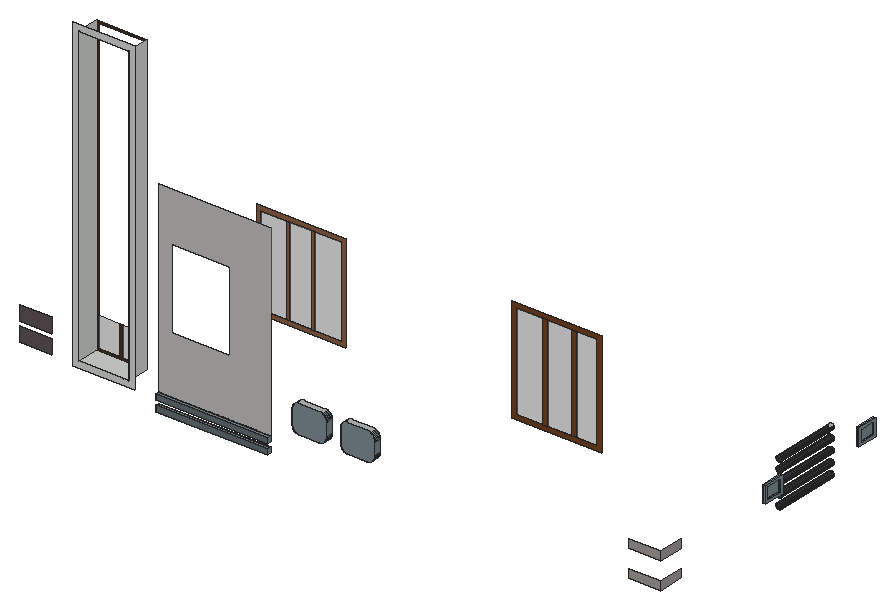
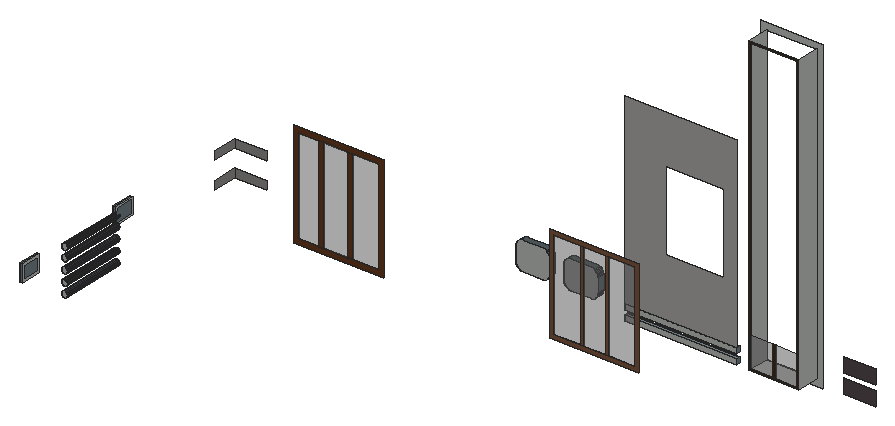
# SketchUp Ruby script. Lengths in inches.
U = 1.inch
M = Sketchup.active_model
def pt(a) = Geom::Point3d.new(a.map { |v| v * U })
def face(e, loops, mat)
  f = e.add_face(loops[0].map { |a| pt(a) })
  loops[1..].each { |l| e.add_face(l.map { |a| pt(a) }).erase! }
  f.material = f.back_material = mat if mat
  f
end
# faces: each face lists its corners as indices into pts; further lists are holes
def faces(e, pts, list, mat = nil) = list.each { |f| face(e, (f[0].is_a?(Array) ? f : [f]).map { |l| l.map { |i| pts[i] } }, mat) }
# xy, xz, yz: faces in a plane at the given z, y or x. An outline is a flat list of corners, or four numbers for a rectangle; further outlines are holes
def ring(l) = l.size == 4 ? [[l[0], l[1]], [l[2], l[1]], [l[2], l[3]], [l[0], l[3]]] : l.each_slice(2).to_a
def flat(e, list, mat, &to3) = list.each { |f| face(e, (f[0].is_a?(Array) ? f : [f]).map { |l| ring(l).map { |u, v| to3.(u, v) } }, mat) }
def xy(e, z, list, mat = nil) = flat(e, list, mat) { |x, y| [x, y, z] }
def xz(e, y, list, mat = nil) = flat(e, list, mat) { |x, z| [x, y, z] }
def yz(e, x, list, mat = nil) = flat(e, list, mat) { |y, z| [x, y, z] }
def lines(e, pts, list) = list.each { |a, b| e.add_line(pt(pts[a]), pt(pts[b])) }
# prism: a flat outline (further loops are holes) pulled along v
def prism(e, loops, v, mat = nil)
  f = face(e, loops, mat); d = Geom::Vector3d.new(v.map { |x| x * U })
  f.pushpull(f.normal.samedirection?(d) ? d.length : -d.length)
end
def box(e, o, s, mat = nil) = prism(e, [[o, [o[0] + s[0], o[1], o[2]], [o[0] + s[0], o[1] + s[1], o[2]], [o[0], o[1] + s[1], o[2]]]], [0, 0, s[2]], mat)
def at(x, y, z, deg = 0) = Geom::Transformation.translation(pt([x, y, z])) * Geom::Transformation.rotation(ORIGIN, Z_AXIS, deg.degrees)
def axes(o, x, y, z) = Geom::Transformation.new([*x, 0, *y, 0, *z, 0, *pt(o).to_a, 1])
def part(name) = M.definitions.add(name)
# library, detail: a bought-in or finely detailed component or shape, given as its bounding box
def library(name, o, s) = part(name).tap { |d| box(d.entities, o, s) }
def detail(e, o, s) = box(e.add_group.entities, o, s)
def put(e, d, t, mat = nil) = e.add_instance(d, t).tap { |i| i.material = mat if mat }
def group(e, t, mat = nil) = e.add_group.tap { |g| g.transformation = t; g.material = mat if mat }.entities
root = M.entities
M.materials.add("[Asphalt New]").color = [89, 79, 82]
M.materials.add("[Basic Tile]").color = [203, 206, 202]
M.materials.add("[Brick Tumbled]").color = [186, 182, 182]
M.materials.add("[Concrete Aggregate Smoke]").color = [154, 150, 148]
M.materials.add("[Formica Laminate Dark]1").color = [65, 69, 79]
M.materials.add("[Formica Speckled Grey]").color = [120, 135, 142]
M.materials.add("[Formica Speckled Grey]1").color = [94, 105, 111]
M.materials.add("[Translucent Glass Gray]").color = [128, 128, 128]
M.materials["[Translucent Glass Gray]"].alpha = 0.5
M.materials.add("[Wood Floor]").color = [71, 48, 28]
M.materials.add("[Wood Veneer 01]1").color = [109, 63, 33]
M.materials.add("[Wood Veneer 02]").color = [137, 92, 65]
xy(root,405.57,[[523.06,696.47,716.67,703.09]],"[Formica Speckled Grey]")
xy(root,414.9375,[[523.06,696.47,716.67,703.09]],"[Formica Speckled Grey]")
xy(root,423.19,[[523.06,696.47,716.67,703.09]],"[Formica Speckled Grey]")
xy(root,432.42,[[385.1,703.09,471.56,741.66]],"[Basic Tile]")
xy(root,432.5625,[[523.06,696.47,716.67,703.09]],"[Formica Speckled Grey]")
xy(root,440.05,[[753.68,719.27,788.14,730.52],[837.48,719.27,870.82,730.52]],"[Formica Speckled Grey]")
xy(root,449.17,[[1370.47,951.61,1374.84,988.05],[1370.47,1153.55,1374.84,1189.99]],"[Formica Speckled Grey]")
xy(root,452.5625,[[1370.47,955.01,1374.84,984.66],[1370.47,1156.95,1374.84,1186.59]],"[Formica Speckled Grey]")
xy(root,474.52,[[1370.47,955.01,1374.84,984.66],[1370.47,1156.95,1374.84,1186.59]],"[Formica Speckled Grey]")
xy(root,477.92,[[1370.47,951.61,1374.84,988.05],[1370.47,1153.55,1374.84,1189.99]],"[Formica Speckled Grey]")
xz(root,696.47,[[523.06,405.57,716.67,414.9375],[523.06,423.19,716.67,432.5625]],"[Formica Speckled Grey]1")
xz(root,703.09,[[282.77,425.33,338.2,450.58],[282.77,458.7,338.2,483.95]],"[Asphalt New]")
xz(root,703.09,[[523.06,405.57,716.67,414.9375],[[374.08,421.4,482.58,954.84],[385.1,432.42,471.56,943.81]],[523.06,423.19,716.67,432.5625]],"[Basic Tile]")
xz(root,703.09,[[[523.06,432.5625,716.67,754.78],[546.1,532.7,646.79,670.32]]],"[Brick Tumbled]")
xz(root,719.27,[[753.68,440.05,788.14,440.05,789.8125,440.16,791.46,440.49,793.05,441.03,794.55,441.77,795.95,442.71,797.21,443.8125,798.32,445.07,799.25,446.47,799.99,447.97,800.53,449.5625,800.86,451.21,800.97,452.88,800.97,476.1,800.86,477.72,800.54,479.31,800.02,480.84,799.31,482.3,798.41,483.64,797.34,484.86,796.12,485.93,794.77,486.83,793.32,487.55,791.78,488.07,790.19,488.39,788.57,488.49,753.6875,488.49,752.04,488.38,750.43,488.0625,748.87,487.53,747.39,486.8,746.02,485.89,744.78,484.8,743.69,483.56,742.78,482.2,742.05,480.72,741.52,479.16,741.2,477.54,741.09,475.9,741.09,452.64,741.2,451,741.52,449.38,742.05,447.82,742.78,446.35,743.69,444.98,744.78,443.74,746.02,442.65,747.38,441.74,748.86,441.01,750.42,440.48,752.03,440.16],[837.48,440.05,870.82,440.05,872.63,440.17,874.42,440.53,876.14,441.11,877.77,441.92,879.28,442.93,880.65,444.125,881.85,445.49,882.86,447,883.66,448.63,884.24,450.36,884.6,452.14,884.72,453.95,884.72,474.16,884.59,476.03,884.23,477.87,883.625,479.64,882.8,481.32,881.76,482.88,880.52,484.29,879.11,485.53,877.55,486.57,875.87,487.4,874.09,488,872.25,488.37,870.38,488.49,837.19,488.49,835.58,488.39,833.99,488.07,832.46,487.55,831.02,486.84,829.67,485.94,828.46,484.875,827.39,483.66,826.5,482.32,825.78,480.87,825.26,479.34,824.95,477.76,824.84,476.14,824.84,452.69,824.95,451.04,825.27,449.42,825.8,447.85,826.53,446.37,827.45,445,828.54,443.76,829.79,442.67,831.16,441.75,832.64,441.02,834.21,440.48,835.83,440.16]],"[Formica Speckled Grey]")
xz(root,730.52,[[753.68,440.05,752.03,440.16,750.42,440.48,748.86,441.01,747.38,441.74,746.02,442.65,744.78,443.74,743.69,444.98,742.78,446.35,742.05,447.82,741.52,449.38,741.2,451,741.09,452.64,741.09,475.9,741.2,477.54,741.52,479.16,742.05,480.72,742.78,482.2,743.69,483.56,744.78,484.8,746.02,485.89,747.39,486.8,748.87,487.53,750.43,488.0625,752.04,488.38,753.6875,488.49,788.57,488.49,790.19,488.39,791.78,488.07,793.32,487.55,794.77,486.83,796.12,485.93,797.34,484.86,798.41,483.64,799.31,482.3,800.02,480.84,800.54,479.31,800.86,477.72,800.97,476.1,800.97,452.88,800.86,451.21,800.53,449.5625,799.99,447.97,799.25,446.47,798.32,445.07,797.21,443.8125,795.95,442.71,794.55,441.77,793.05,441.03,791.46,440.49,789.8125,440.16,788.14,440.05],[837.48,440.05,835.83,440.16,834.21,440.48,832.64,441.02,831.16,441.75,829.79,442.67,828.54,443.76,827.45,445,826.53,446.37,825.8,447.85,825.27,449.42,824.95,451.04,824.84,452.69,824.84,476.14,824.95,477.76,825.26,479.34,825.78,480.87,826.5,482.32,827.39,483.66,828.46,484.875,829.67,485.94,831.02,486.84,832.46,487.55,833.99,488.07,835.58,488.39,837.19,488.49,870.38,488.49,872.25,488.37,874.09,488,875.87,487.4,877.55,486.57,879.11,485.53,880.52,484.29,881.76,482.88,882.8,481.32,883.625,479.64,884.23,477.87,884.59,476.03,884.72,474.16,884.72,453.95,884.6,452.14,884.24,450.36,883.66,448.63,882.86,447,881.85,445.49,880.65,444.125,879.28,442.93,877.77,441.92,876.14,441.11,874.42,440.53,872.63,440.17,870.82,440.05]],"[Basic Tile]")
xz(root,730.52,[[1314.99,410.47,1370.47,425.22],[1314.99,456.66,1370.47,471.41]],"[Concrete Aggregate Smoke]")
xz(root,741.66,[[387.85,435.17,425.21,487.63],[430.65,435.17,468.81,487.63]],"[Translucent Glass Gray]")
xz(root,741.66,[[[385.1,432.42,471.56,943.81],[387.85,435.17,468.81,941.07]],[425.21,435.17,430.65,487.63]],"[Wood Floor]")
xz(root,898.23,[[987.57,475.01,1032.05,640.23],[1039.98,475.01,1082.49,640.23],[1090.42,475.01,1125.29,640.23],[544.07,481.83,588.26,635.98],[594.65,481.83,631.26,635.98],
  [637.65,481.83,683.83,635.98]],"[Translucent Glass Gray]")
xz(root,898.23,[[[978.99,466.43,1133.86,648.81],[987.57,475.01,1125.29,640.23]],[1032.05,475.01,1039.98,640.23],[1082.49,475.01,1090.42,640.23]],"[Wood Veneer 01]1")
xz(root,898.23,[[[536.84,474.6,691.07,643.21],[544.07,481.83,683.83,635.98]],[588.26,481.83,594.65,635.98],[631.26,481.83,637.65,635.98]],"[Wood Veneer 02]")
xz(root,951.61,[[1370.47,449.17,1374.84,477.92]],"[Formica Speckled Grey]")
xz(root,955.01,[[1370.47,452.5625,1374.84,474.52]],"[Formica Speckled Grey]")
xz(root,984.66,[[1370.47,452.5625,1374.84,474.52]],"[Formica Speckled Grey]")
xz(root,988.05,[[1370.47,449.17,1374.84,477.92]],"[Formica Speckled Grey]")
xz(root,1125.19,[[1349.2,405.1,1347.875,405.28,1346.64,405.79,1345.58,406.61,1344.76,407.67,1344.25,408.9,1344.08,410.23,1344.25,411.56,1344.76,412.79,1345.58,413.85,1346.64,414.67,1347.875,415.18,1349.2,415.35,1350.53,415.18,1351.77,414.67,1352.83,413.85,1353.64,412.79,1354.15,411.56,1354.33,410.23,1354.15,408.9,1353.64,407.67,1352.83,406.61,1351.77,405.79,1350.53,405.28],[1349.2,423.29,1347.875,423.47,1346.64,423.98,1345.58,424.79,1344.76,425.85,1344.25,427.09,1344.08,428.42,1344.25,429.74,1344.76,430.98,1345.58,432.04,1346.64,432.86,1347.875,433.37,1349.2,433.54,1350.53,433.37,1351.77,432.86,1352.83,432.04,1353.64,430.98,1354.15,429.74,1354.33,428.42,1354.15,427.09,1353.64,425.85,1352.83,424.79,1351.77,423.98,1350.53,423.47],[1349.2,442.67,1347.875,442.84,1346.64,443.35,1345.58,444.17,1344.76,445.23,1344.25,446.47,1344.08,447.79,1344.25,449.12,1344.76,450.35,1345.58,451.42,1346.64,452.23,1347.875,452.74,1349.2,452.92,1350.53,452.74,1351.77,452.23,1352.83,451.42,1353.64,450.35,1354.15,449.12,1354.33,447.79,1354.15,446.47,1353.64,445.23,1352.83,444.17,1351.77,443.35,1350.53,442.84],[1349.2,461.48,1347.875,461.65,1346.64,462.17,1345.58,462.98,1344.76,464.04,1344.25,465.28,1344.08,466.6,1344.25,467.93,1344.76,469.17,1345.58,470.23,1346.64,471.04,1347.875,471.55,1349.2,471.73,1350.53,471.55,1351.77,471.04,1352.83,470.23,1353.64,469.17,1354.15,467.93,1354.33,466.6,1354.15,465.28,1353.64,464.04,1352.83,462.98,1351.77,462.17,1350.53,461.65],[1349.2,478.79,1347.875,478.97,1346.64,479.48,1345.58,480.29,1344.76,481.35,1344.25,482.59,1344.08,483.92,1344.25,485.24,1344.76,486.48,1345.58,487.54,1346.64,488.36,1347.875,488.87,1349.2,489.04,1350.53,488.87,1351.77,488.36,1352.83,487.54,1353.64,486.48,1354.15,485.24,1354.33,483.92,1354.15,482.59,1353.64,481.35,1352.83,480.29,1351.77,479.48,1350.53,478.97]],"[Basic Tile]")
xz(root,1153.55,[[1370.47,449.17,1374.84,477.92]],"[Formica Speckled Grey]")
xz(root,1156.95,[[1370.47,452.5625,1374.84,474.52]],"[Formica Speckled Grey]")
xz(root,1186.59,[[1370.47,452.5625,1374.84,474.52]],"[Formica Speckled Grey]")
xz(root,1189.99,[[1370.47,449.17,1374.84,477.92]],"[Formica Speckled Grey]")
yz(root,385.1,[[703.09,432.42,741.66,943.81]],"[Basic Tile]")
yz(root,471.56,[[703.09,432.42,741.66,943.81]],"[Basic Tile]")
yz(root,523.06,[[696.47,405.57,703.09,414.9375],[696.47,423.19,703.09,432.5625]],"[Formica Speckled Grey]")
yz(root,716.67,[[696.47,405.57,703.09,414.9375],[696.47,423.19,703.09,432.5625]],"[Formica Speckled Grey]")
yz(root,741.09,[[719.27,452.64,730.52,475.9]],"[Formica Speckled Grey]")
yz(root,800.97,[[719.27,452.88,730.52,476.1]],"[Formica Speckled Grey]")
yz(root,824.84,[[719.27,452.69,730.52,476.14]],"[Formica Speckled Grey]")
yz(root,884.72,[[719.27,453.95,730.52,474.16]],"[Formica Speckled Grey]")
yz(root,1370.47,[[[951.61,449.17,988.05,477.92],[955.01,452.5625,984.66,474.52]],[[1153.55,449.17,1189.99,477.92],[1156.95,452.5625,1186.59,474.52]]],"[Basic Tile]")
yz(root,1370.47,[[730.52,410.47,774.21,425.22],[730.52,456.66,774.21,471.41]],"[Concrete Aggregate Smoke]")
yz(root,1370.47,[[955.01,452.5625,984.66,474.52],[1156.95,452.5625,1186.59,474.52]],"[Formica Speckled Grey]")
yz(root,1374.84,[[[951.61,449.17,988.05,477.92],[955.01,452.5625,984.66,474.52]],[[1153.55,449.17,1189.99,477.92],[1156.95,452.5625,1186.59,474.52]]],"[Formica Speckled Grey]")
p = [[1347.875,1125.19,405.28],[1349.2,1125.19,405.1],[1349.2,1012.73,405.1],[1347.875,1012.73,405.28],[1350.53,1125.19,405.28],[1350.53,1012.73,405.28],
  [1346.64,1125.19,405.79],[1346.64,1012.73,405.79],[1351.77,1125.19,405.79],[1351.77,1012.73,405.79],[1345.58,1125.19,406.61],[1345.58,1012.73,406.61],
  [1352.83,1125.19,406.61],[1352.83,1012.73,406.61],[1344.76,1125.19,407.67],[1344.76,1012.73,407.67],[1353.64,1125.19,407.67],[1353.64,1012.73,407.67],
  [1344.25,1125.19,408.9],[1344.25,1012.73,408.9],[1354.15,1125.19,408.9],[1354.15,1012.73,408.9],[1344.08,1125.19,410.23],[1344.08,1012.73,410.23],
  [1354.33,1125.19,410.23],[1354.33,1012.73,410.23],[1344.25,1125.19,411.56],[1344.25,1012.73,411.56],[1354.15,1125.19,411.56],[1354.15,1012.73,411.56],
  [1344.76,1125.19,412.79],[1344.76,1012.73,412.79],[1353.64,1125.19,412.79],[1353.64,1012.73,412.79],[1345.58,1125.19,413.85],[1345.58,1012.73,413.85],
  [1352.83,1125.19,413.85],[1352.83,1012.73,413.85],[1346.64,1125.19,414.67],[1346.64,1012.73,414.67],[1351.77,1125.19,414.67],[1351.77,1012.73,414.67],
  [1347.875,1125.19,415.18],[1347.875,1012.73,415.18],[1350.53,1125.19,415.18],[1350.53,1012.73,415.18],[1349.2,1125.19,415.35],[1349.2,1012.73,415.35],
  [1347.875,1125.19,423.47],[1349.2,1125.19,423.29],[1349.2,1012.73,423.29],[1347.875,1012.73,423.47],[1350.53,1125.19,423.47],[1350.53,1012.73,423.47],
  [1346.64,1125.19,423.98],[1346.64,1012.73,423.98],[1351.77,1125.19,423.98],[1351.77,1012.73,423.98],[1345.58,1125.19,424.79],[1345.58,1012.73,424.79],
  [1352.83,1125.19,424.79],[1352.83,1012.73,424.79],[1344.76,1125.19,425.85],[1344.76,1012.73,425.85],[1353.64,1125.19,425.85],[1353.64,1012.73,425.85],
  [1344.25,1125.19,427.09],[1344.25,1012.73,427.09],[1354.15,1125.19,427.09],[1354.15,1012.73,427.09],[1344.08,1125.19,428.42],[1344.08,1012.73,428.42],
  [1354.33,1125.19,428.42],[1354.33,1012.73,428.42],[1344.25,1125.19,429.74],[1344.25,1012.73,429.74],[1354.15,1125.19,429.74],[1354.15,1012.73,429.74],
  [1344.76,1125.19,430.98],[1344.76,1012.73,430.98],[1353.64,1125.19,430.98],[1353.64,1012.73,430.98],[1345.58,1125.19,432.04],[1345.58,1012.73,432.04],
  [1352.83,1125.19,432.04],[1352.83,1012.73,432.04],[1346.64,1125.19,432.86],[1346.64,1012.73,432.86],[1351.77,1125.19,432.86],[1351.77,1012.73,432.86],
  [1347.875,1125.19,433.37],[1347.875,1012.73,433.37],[1350.53,1125.19,433.37],[1350.53,1012.73,433.37],[1349.2,1125.19,433.54],[1349.2,1012.73,433.54],
  [752.03,730.52,440.16],[753.68,730.52,440.05],[753.68,719.27,440.05],[752.03,719.27,440.16],[788.14,730.52,440.05],[789.8125,730.52,440.16],
  [789.8125,719.27,440.16],[788.14,719.27,440.05],[835.83,730.52,440.16],[837.48,730.52,440.05],[837.48,719.27,440.05],[835.83,719.27,440.16],
  [870.82,730.52,440.05],[872.63,730.52,440.17],[872.63,719.27,440.17],[870.82,719.27,440.05],[750.42,730.52,440.48],[750.42,719.27,440.48],
  [791.46,730.52,440.49],[791.46,719.27,440.49],[834.21,730.52,440.48],[834.21,719.27,440.48],[874.42,730.52,440.53],[874.42,719.27,440.53],
  [748.86,730.52,441.01],[748.86,719.27,441.01],[793.05,730.52,441.03],[793.05,719.27,441.03],[832.64,730.52,441.02],[832.64,719.27,441.02],
  [876.14,730.52,441.11],[876.14,719.27,441.11],[747.38,730.52,441.74],[747.38,719.27,441.74],[794.55,730.52,441.77],[794.55,719.27,441.77],
  [831.16,730.52,441.75],[831.16,719.27,441.75],[877.77,730.52,441.92],[877.77,719.27,441.92],[746.02,730.52,442.65],[746.02,719.27,442.65],
  [829.79,730.52,442.67],[829.79,719.27,442.67],[795.95,730.52,442.71],[795.95,719.27,442.71],[879.28,730.52,442.93],[879.28,719.27,442.93],
  [744.78,730.52,443.74],[744.78,719.27,443.74],[797.21,730.52,443.8125],[797.21,719.27,443.8125],[828.54,730.52,443.76],[828.54,719.27,443.76],
  [1347.875,1125.19,442.84],[1349.2,1125.19,442.67],[1349.2,1012.73,442.67],[1347.875,1012.73,442.84],[1350.53,1125.19,442.84],[1350.53,1012.73,442.84],
  [1346.64,1125.19,443.35],[1346.64,1012.73,443.35],[1351.77,1125.19,443.35],[1351.77,1012.73,443.35],[880.65,730.52,444.125],[880.65,719.27,444.125],
  [1345.58,1125.19,444.17],[1345.58,1012.73,444.17],[1352.83,1125.19,444.17],[1352.83,1012.73,444.17],[743.69,730.52,444.98],[743.69,719.27,444.98],
  [798.32,730.52,445.07],[798.32,719.27,445.07],[827.45,730.52,445],[827.45,719.27,445],[881.85,730.52,445.49],[881.85,719.27,445.49],
  [1344.76,1125.19,445.23],[1344.76,1012.73,445.23],[1353.64,1125.19,445.23],[1353.64,1012.73,445.23],[742.78,730.52,446.35],[742.78,719.27,446.35],
  [826.53,730.52,446.37],[826.53,719.27,446.37],[799.25,730.52,446.47],[799.25,719.27,446.47],[1344.25,1125.19,446.47],[1344.25,1012.73,446.47],
  [1354.15,1125.19,446.47],[1354.15,1012.73,446.47],[882.86,730.52,447],[882.86,719.27,447],[742.05,730.52,447.82],[742.05,719.27,447.82],
  [825.8,730.52,447.85],[825.8,719.27,447.85],[799.99,730.52,447.97],[799.99,719.27,447.97],[1344.08,1125.19,447.79],[1344.08,1012.73,447.79],
  [1354.33,1125.19,447.79],[1354.33,1012.73,447.79],[883.66,730.52,448.63],[883.66,719.27,448.63],[741.52,730.52,449.38],[741.52,719.27,449.38],
  [1344.25,1125.19,449.12],[1344.25,1012.73,449.12],[1354.15,1125.19,449.12],[1354.15,1012.73,449.12],[825.27,730.52,449.42],[825.27,719.27,449.42],
  [800.53,730.52,449.5625],[800.53,719.27,449.5625],[884.24,730.52,450.36],[884.24,719.27,450.36],[1344.76,1125.19,450.35],[1344.76,1012.73,450.35],
  [1353.64,1125.19,450.35],[1353.64,1012.73,450.35],[741.2,730.52,451],[741.2,719.27,451],[824.95,730.52,451.04],[824.95,719.27,451.04],
  [800.86,730.52,451.21],[800.86,719.27,451.21],[884.6,730.52,452.14],[884.6,719.27,452.14],[1345.58,1125.19,451.42],[1345.58,1012.73,451.42],
  [1352.83,1125.19,451.42],[1352.83,1012.73,451.42],[741.09,730.52,452.64],[741.09,719.27,452.64],[824.84,730.52,452.69],[824.84,719.27,452.69],
  [800.97,730.52,452.88],[800.97,719.27,452.88],[1346.64,1125.19,452.23],[1346.64,1012.73,452.23],[1351.77,1125.19,452.23],[1351.77,1012.73,452.23],
  [884.72,730.52,453.95],[884.72,719.27,453.95],[1347.875,1125.19,452.74],[1347.875,1012.73,452.74],[1350.53,1125.19,452.74],[1350.53,1012.73,452.74],
  [1349.2,1125.19,452.92],[1349.2,1012.73,452.92],[1347.875,1125.19,461.65],[1349.2,1125.19,461.48],[1349.2,1012.73,461.48],[1347.875,1012.73,461.65],
  [1350.53,1125.19,461.65],[1350.53,1012.73,461.65],[1346.64,1125.19,462.17],[1346.64,1012.73,462.17],[1351.77,1125.19,462.17],[1351.77,1012.73,462.17],
  [1345.58,1125.19,462.98],[1345.58,1012.73,462.98],[1352.83,1125.19,462.98],[1352.83,1012.73,462.98],[1344.76,1125.19,464.04],[1344.76,1012.73,464.04],
  [1353.64,1125.19,464.04],[1353.64,1012.73,464.04],[1344.25,1125.19,465.28],[1344.25,1012.73,465.28],[1354.15,1125.19,465.28],[1354.15,1012.73,465.28],
  [1344.08,1125.19,466.6],[1344.08,1012.73,466.6],[1354.33,1125.19,466.6],[1354.33,1012.73,466.6],[1344.25,1125.19,467.93],[1344.25,1012.73,467.93],
  [1354.15,1125.19,467.93],[1354.15,1012.73,467.93],[1344.76,1125.19,469.17],[1344.76,1012.73,469.17],[1353.64,1125.19,469.17],[1353.64,1012.73,469.17],
  [1345.58,1125.19,470.23],[1345.58,1012.73,470.23],[1352.83,1125.19,470.23],[1352.83,1012.73,470.23],[1346.64,1125.19,471.04],[1346.64,1012.73,471.04],
  [1351.77,1125.19,471.04],[1351.77,1012.73,471.04],[1347.875,1125.19,471.55],[1347.875,1012.73,471.55],[1350.53,1125.19,471.55],[1350.53,1012.73,471.55],
  [1349.2,1125.19,471.73],[1349.2,1012.73,471.73],[884.72,730.52,474.16],[884.59,730.52,476.03],[884.59,719.27,476.03],[884.72,719.27,474.16],
  [741.2,730.52,477.54],[741.09,730.52,475.9],[741.09,719.27,475.9],[741.2,719.27,477.54],[884.23,730.52,477.87],[884.23,719.27,477.87],
  [800.97,730.52,476.1],[800.86,730.52,477.72],[800.86,719.27,477.72],[800.97,719.27,476.1],[824.95,730.52,477.76],[824.84,730.52,476.14],
  [824.84,719.27,476.14],[824.95,719.27,477.76],[741.52,730.52,479.16],[741.52,719.27,479.16],[800.54,730.52,479.31],[800.54,719.27,479.31],
  [825.26,730.52,479.34],[825.26,719.27,479.34],[883.625,730.52,479.64],[883.625,719.27,479.64],[1347.875,1125.19,478.97],[1349.2,1125.19,478.79],
  [1349.2,1012.73,478.79],[1347.875,1012.73,478.97],[1350.53,1125.19,478.97],[1350.53,1012.73,478.97],[1346.64,1125.19,479.48],[1346.64,1012.73,479.48],
  [1351.77,1125.19,479.48],[1351.77,1012.73,479.48],[742.05,730.52,480.72],[742.05,719.27,480.72],[800.02,730.52,480.84],[800.02,719.27,480.84],
  [825.78,730.52,480.87],[825.78,719.27,480.87],[1345.58,1125.19,480.29],[1345.58,1012.73,480.29],[1352.83,1125.19,480.29],[1352.83,1012.73,480.29],
  [882.8,730.52,481.32],[882.8,719.27,481.32],[1344.76,1125.19,481.35],[1344.76,1012.73,481.35],[1353.64,1125.19,481.35],[1353.64,1012.73,481.35],
  [742.78,730.52,482.2],[742.78,719.27,482.2],[799.31,730.52,482.3],[799.31,719.27,482.3],[826.5,730.52,482.32],[826.5,719.27,482.32],
  [881.76,730.52,482.88],[881.76,719.27,482.88],[1344.25,1125.19,482.59],[1344.25,1012.73,482.59],[1354.15,1125.19,482.59],[1354.15,1012.73,482.59],
  [743.69,730.52,483.56],[743.69,719.27,483.56],[798.41,730.52,483.64],[798.41,719.27,483.64],[827.39,730.52,483.66],[827.39,719.27,483.66],
  [1344.08,1125.19,483.92],[1344.08,1012.73,483.92],[1354.33,1125.19,483.92],[1354.33,1012.73,483.92],[880.52,730.52,484.29],[880.52,719.27,484.29],
  [744.78,730.52,484.8],[744.78,719.27,484.8],[797.34,730.52,484.86],[797.34,719.27,484.86],[828.46,730.52,484.875],[828.46,719.27,484.875],
  [1344.25,1125.19,485.24],[1344.25,1012.73,485.24],[1354.15,1125.19,485.24],[1354.15,1012.73,485.24],[879.11,730.52,485.53],[879.11,719.27,485.53],
  [746.02,730.52,485.89],[746.02,719.27,485.89],[796.12,730.52,485.93],[796.12,719.27,485.93],[829.67,730.52,485.94],[829.67,719.27,485.94],
  [1344.76,1125.19,486.48],[1344.76,1012.73,486.48],[1353.64,1125.19,486.48],[1353.64,1012.73,486.48],[877.55,730.52,486.57],[877.55,719.27,486.57],
  [747.39,730.52,486.8],[747.39,719.27,486.8],[794.77,730.52,486.83],[794.77,719.27,486.83],[831.02,730.52,486.84],[831.02,719.27,486.84]]
faces(root,p,[[0,1,2,3],[1,4,5,2],[6,0,3,7],[4,8,9,5],[10,6,7,11],[8,12,13,9],[14,10,11,15],[12,16,17,13],
  [18,14,15,19],[16,20,21,17],[22,18,19,23],[20,24,25,21],[26,22,23,27],[24,28,29,25],[30,26,27,31],[28,32,33,29],
  [34,30,31,35],[32,36,37,33],[38,34,35,39],[36,40,41,37],[42,38,39,43],[40,44,45,41],[46,42,43,47],[44,46,47,45],
  [48,49,50,51],[49,52,53,50],[54,48,51,55],[52,56,57,53],[58,54,55,59],[56,60,61,57],[62,58,59,63],[60,64,65,61],
  [66,62,63,67],[64,68,69,65],[70,66,67,71],[68,72,73,69],[74,70,71,75],[72,76,77,73],[78,74,75,79],[76,80,81,77],
  [82,78,79,83],[80,84,85,81],[86,82,83,87],[84,88,89,85],[90,86,87,91],[88,92,93,89],[94,90,91,95],[92,94,95,93],
  [150,151,152,153],[151,154,155,152],[156,150,153,157],[154,158,159,155],[162,156,157,163],[158,164,165,159],[174,162,163,175],[164,176,177,165],
  [184,174,175,185],[176,186,187,177],[196,184,185,197],[186,198,199,187],[204,196,197,205],[198,206,207,199],[214,204,205,215],[206,216,217,207],
  [226,214,215,227],[216,228,229,217],[236,226,227,237],[228,238,239,229],[242,236,237,243],[238,244,245,239],[246,242,243,247],[244,246,247,245],
  [248,249,250,251],[249,252,253,250],[254,248,251,255],[252,256,257,253],[258,254,255,259],[256,260,261,257],[262,258,259,263],[260,264,265,261],
  [266,262,263,267],[264,268,269,265],[270,266,267,271],[268,272,273,269],[274,270,271,275],[272,276,277,273],[278,274,275,279],[276,280,281,277],
  [282,278,279,283],[280,284,285,281],[286,282,283,287],[284,288,289,285],[290,286,287,291],[288,292,293,289],[294,290,291,295],[292,294,295,293],
  [322,323,324,325],[323,326,327,324],[328,322,325,329],[326,330,331,327],[338,328,329,339],[330,340,341,331],[344,338,339,345],[340,346,347,341],
  [356,344,345,357],[346,358,359,347],[366,356,357,367],[358,368,369,359],[378,366,367,379],[368,380,381,369],[390,378,379,391],[380,392,393,381]],"[Formica Laminate Dark]1")
faces(root,p,[[96,97,98,99],[100,101,102,103],[104,105,106,107],[108,109,110,111],[112,96,99,113],[101,114,115,102],[116,104,107,117],[109,118,119,110],
  [120,112,113,121],[114,122,123,115],[124,116,117,125],[118,126,127,119],[128,120,121,129],[122,130,131,123],[132,124,125,133],[126,134,135,127],
  [136,128,129,137],[138,132,133,139],[130,140,141,131],[134,142,143,135],[144,136,137,145],[140,146,147,141],[148,138,139,149],[142,160,161,143],
  [166,144,145,167],[146,168,169,147],[170,148,149,171],[160,172,173,161],[178,166,167,179],[180,170,171,181],[168,182,183,169],[172,188,189,173],
  [190,178,179,191],[192,180,181,193],[182,194,195,183],[188,200,201,189],[202,190,191,203],[208,192,193,209],[194,210,211,195],[200,212,213,201],
  [218,202,203,219],[220,208,209,221],[210,222,223,211],[212,224,225,213],[230,218,219,231],[232,220,221,233],[222,234,235,223],[224,240,241,225],
  [296,297,298,299],[300,301,302,303],[297,304,305,298],[306,307,308,309],[310,311,312,313],[314,300,303,315],[307,316,317,308],[318,310,313,319],
  [304,320,321,305],[332,314,315,333],[316,334,335,317],[336,318,319,337],[320,342,343,321],[348,332,333,349],[334,350,351,335],[352,336,337,353],
  [342,354,355,343],[360,348,349,361],[350,362,363,351],[364,352,353,365],[354,370,371,355],[372,360,361,373],[362,374,375,363],[376,364,365,377],
  [370,382,383,371],[384,372,373,385],[374,386,387,375],[388,376,377,389],[382,394,395,383],[396,384,385,397],[386,398,399,387],[400,388,389,401]],"[Formica Speckled Grey]")
